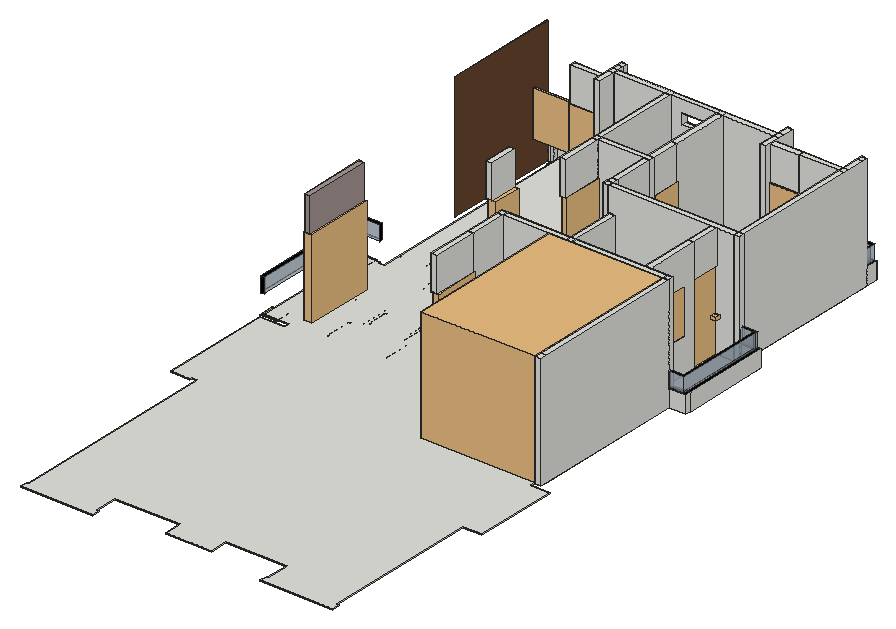
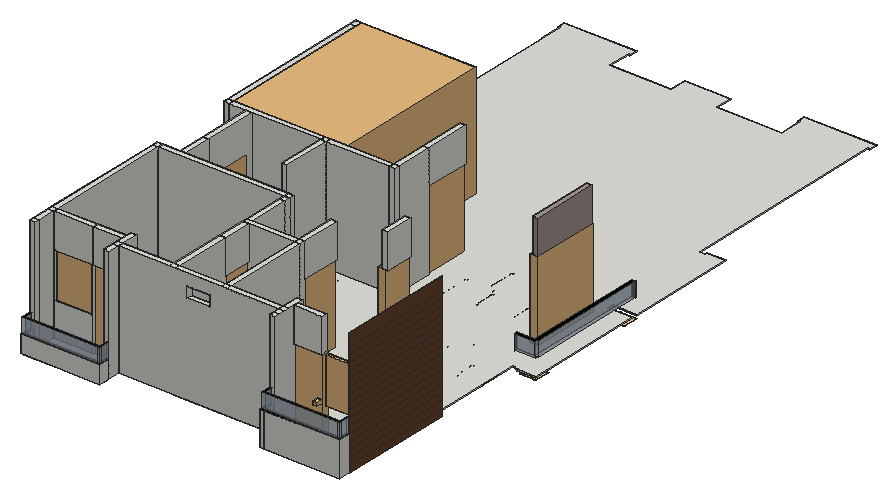
# SketchUp Ruby script. Lengths in inches.
U = 1.inch
M = Sketchup.active_model
def pt(a) = Geom::Point3d.new(a.map { |v| v * U })
def face(e, loops, mat)
  f = e.add_face(loops[0].map { |a| pt(a) })
  loops[1..].each { |l| e.add_face(l.map { |a| pt(a) }).erase! }
  f.material = f.back_material = mat if mat
  f
end
# faces: each face lists its corners as indices into pts; further lists are holes
def faces(e, pts, list, mat = nil) = list.each { |f| face(e, (f[0].is_a?(Array) ? f : [f]).map { |l| l.map { |i| pts[i] } }, mat) }
# xy, xz, yz: faces in a plane at the given z, y or x. An outline is a flat list of corners, or four numbers for a rectangle; further outlines are holes
def ring(l) = l.size == 4 ? [[l[0], l[1]], [l[2], l[1]], [l[2], l[3]], [l[0], l[3]]] : l.each_slice(2).to_a
def flat(e, list, mat, &to3) = list.each { |f| face(e, (f[0].is_a?(Array) ? f : [f]).map { |l| ring(l).map { |u, v| to3.(u, v) } }, mat) }
def xy(e, z, list, mat = nil) = flat(e, list, mat) { |x, y| [x, y, z] }
def xz(e, y, list, mat = nil) = flat(e, list, mat) { |x, z| [x, y, z] }
def yz(e, x, list, mat = nil) = flat(e, list, mat) { |y, z| [x, y, z] }
def lines(e, pts, list) = list.each { |a, b| e.add_line(pt(pts[a]), pt(pts[b])) }
# prism: a flat outline (further loops are holes) pulled along v
def prism(e, loops, v, mat = nil)
  f = face(e, loops, mat); d = Geom::Vector3d.new(v.map { |x| x * U })
  f.pushpull(f.normal.samedirection?(d) ? d.length : -d.length)
end
def box(e, o, s, mat = nil) = prism(e, [[o, [o[0] + s[0], o[1], o[2]], [o[0] + s[0], o[1] + s[1], o[2]], [o[0], o[1] + s[1], o[2]]]], [0, 0, s[2]], mat)
def at(x, y, z, deg = 0) = Geom::Transformation.translation(pt([x, y, z])) * Geom::Transformation.rotation(ORIGIN, Z_AXIS, deg.degrees)
def axes(o, x, y, z) = Geom::Transformation.new([*x, 0, *y, 0, *z, 0, *pt(o).to_a, 1])
def part(name) = M.definitions.add(name)
# library, detail: a bought-in or finely detailed component or shape, given as its bounding box
def library(name, o, s) = part(name).tap { |d| box(d.entities, o, s) }
def detail(e, o, s) = box(e.add_group.entities, o, s)
def put(e, d, t, mat = nil) = e.add_instance(d, t).tap { |i| i.material = mat if mat }
def group(e, t, mat = nil) = e.add_group.tap { |g| g.transformation = t; g.material = mat if mat }.entities
root = M.entities
M.materials.add("0-off white").color = [255, 255, 255]
M.materials.add("Glass_Basic_01").color = [161, 173, 186]
M.materials["Glass_Basic_01"].alpha = 0.59
M.materials.add("M09_Shadow_Night").color = [0, 0, 0]
M.materials.add("Marble_06_1K").color = [165, 150, 147]
M.materials.add("Wood_Veneer_15_1K").color = [103, 69, 45]
c1 = library("Return staircase",[0,-11.89,0],[120,168,120])
c2 = part("Group\#84")
xy(c2.entities,0,[[[-2,-32,-2,-24,0.04,-24,0.04,0,0,0,0,198,-6,198,-6,196,-25.9,196,-25.9,312.57,0,312.57,0,318.21,-25.9,318.21,-25.9,446,-6,446,-6,444,0,444,0,675.78,72,673.93,76,673.93,76,665.93,74,665.93,74,636,252.4,636,252.4,673.93,328.4,673.93,328.4,636,324.4,636,324.4,498.14,330.4,498.14,330.4,499.84,344.35,499.84,344.35,411,324.4,411,324.4,231,344.35,231,344.35,142,324.4,142,324.4,0,324.58,0,324.58,-24,326.4,-24,326.4,-32,250.4,-32,250.4,-24,252.4,-24,252.4,0,188.4,0,188.4,-18,140,-18,140,0,72,0,72,-24,74,-24,74,-32],[210.4,291,270.4,351]]])
xy(c2.entities,1,[[[-2,-32,74,-32,74,-24,72,-24,72,0,140,0,140,-18,188.4,-18,188.4,0,252.4,0,252.4,-24,250.4,-24,250.4,-32,326.4,-32,326.4,-24,324.58,-24,324.58,0,324.4,0,324.4,142,344.35,142,344.35,231,324.4,231,324.4,411,344.35,411,344.35,499.84,330.4,499.84,330.4,498.14,324.4,498.14,324.4,636,328.4,636,328.4,673.93,252.4,673.93,252.4,636,74,636,74,665.93,76,665.93,76,673.93,72,673.93,0,675.78,0,444,-6,444,-6,446,-25.9,446,-25.9,318.21,0,318.21,0,312.57,-25.9,312.57,-25.9,196,-6,196,-6,198,0,198,0,0,0.04,0,0.04,-24,-2,-24],[210.4,291,270.4,351]]])
xz(c2.entities,-32,[[-2,0,74,1],[250.4,0,326.4,1]])
xz(c2.entities,-24,[[-2,0,0.04,1],[72,0,74,1],[250.4,0,252.4,1],[324.58,0,326.4,1]])
xz(c2.entities,-18,[[140,0,188.4,1]])
xz(c2.entities,0,[[0,0,0.04,1],[72,0,140,1],[188.4,0,252.4,1],[324.4,0,324.58,1]])
xz(c2.entities,142,[[324.4,0,344.35,1]])
xz(c2.entities,196,[[-25.9,0,-6,1]])
xz(c2.entities,198,[[-6,0,0,1]])
xz(c2.entities,231,[[324.4,0,344.35,1]])
xz(c2.entities,291,[[210.4,0,270.4,1]])
xz(c2.entities,312.57,[[-25.9,0,0,1]])
xz(c2.entities,318.21,[[-25.9,0,0,1]])
xz(c2.entities,351,[[210.4,0,270.4,1]])
xz(c2.entities,411,[[324.4,0,344.35,1]])
xz(c2.entities,444,[[-6,0,0,1]])
xz(c2.entities,446,[[-25.9,0,-6,1]])
xz(c2.entities,498.14,[[324.4,0,330.4,1]])
xz(c2.entities,499.84,[[330.4,0,344.35,1]])
xz(c2.entities,636,[[74,0,252.4,1],[324.4,0,328.4,1]])
xz(c2.entities,665.93,[[74,0,76,1]])
xz(c2.entities,673.93,[[72,0,76,1],[252.4,0,328.4,1]])
yz(c2.entities,-25.9,[[196,0,312.57,1],[318.21,0,446,1]])
yz(c2.entities,-6,[[196,0,198,1],[444,0,446,1]])
yz(c2.entities,-2,[[-32,0,-24,1]])
yz(c2.entities,0,[[0,0,198,1],[312.57,0,318.21,1],[444,0,636,1],[636,0,637.85,1],[637.85,0,675.78,1]])
yz(c2.entities,0.04,[[-24,0,0,1]])
yz(c2.entities,72,[[-24,0,0,1]])
yz(c2.entities,74,[[-32,0,-24,1],[636,0,665.93,1]])
yz(c2.entities,76,[[665.93,0,673.93,1]])
yz(c2.entities,140,[[-18,0,0,1]])
yz(c2.entities,188.4,[[-18,0,0,1]])
yz(c2.entities,210.4,[[291,0,351,1]])
yz(c2.entities,250.4,[[-32,0,-24,1]])
yz(c2.entities,252.4,[[-24,0,0,1],[636,0,673.93,1]])
yz(c2.entities,270.4,[[291,0,351,1]])
yz(c2.entities,324.4,[[0,0,142,1],[231,0,411,1],[498.14,0,636,1]])
yz(c2.entities,324.58,[[-24,0,0,1]])
yz(c2.entities,326.4,[[-32,0,-24,1]])
yz(c2.entities,328.4,[[636,0,673.93,1]])
yz(c2.entities,330.4,[[498.14,0,499.84,1]])
yz(c2.entities,344.35,[[142,0,231,1],[411,0,499.84,1]])
# 3 loose lines left out
p = [[77.67,648,0],[77.67,636,1],[246.4,636,1],[246.4,648,0],[72,673.93,0],[0,675.78,0],
  [0,675.78,1],[72,673.93,1]]
faces(c2.entities,p,[[0,1,2,3],[4,5,6,7]])
c3 = library("TREE-26",[-60.96,-72.91,0],[121.92,134.74,0.01])
c4 = library("HYHHYHYHYHYHY",[-2.09,-4.54,0],[4.18,9.08,0.01])
c5 = library("Group\#51",[0,0,0],[6.9375,42,86.5])
c6 = part("feeeeeeeeee")
p = [[-2.68,3.51,0],[-2.68,3.16,0],[-2.92,3.16,0],[-2.92,3.07,0],[-3.56,3.07,0],[-3.56,3.51,0],
  [-2.68,-3.51,0],[-2.68,-3.16,0],[-2.92,-3.16,0],[-2.92,-3.07,0],[-3.56,-3.07,0],[-3.56,-3.51,0],
  [3.56,3.16,0],[-2.68,2.93,0],[3.56,2.93,0],[-2.48,-3.13,0],[-2.04,-3.07,0],[-1.61,-2.98,0],
  [-1.1875,-2.86,0],[-0.77,-2.72,0],[-0.36,-2.55,0],[0.03,-2.35,0],[0.41,-2.13,0],[0.78,-1.88,0],
  [1.125,-1.62,0],[1.46,-1.32,0],[1.77,-1.01,0],[2.06,-0.68,0],[2.33,-0.33,0],[2.57,0.03,0],
  [2.79,0.42,0],[2.99,0.81,0],[3.16,1.22,0],[3.3,1.63,0],[3.41,2.06,0],[3.5,2.49,0]]
lines(c6.entities,p,[[0,1],[1,2],[2,3],[3,4],[4,5],[5,0],[6,7],[7,8],[8,9],[9,10],[10,11],[11,6],
  [1,12],[13,14],[1,13],[12,14],[8,15],[15,16],[16,17],[17,18],[18,19],[19,20],[20,21],[21,22],
  [22,23],[23,24],[24,25],[25,26],[26,27],[27,28],[28,29],[29,30],[30,31],[31,32],[32,33],[33,34],
  [34,35],[35,14]])
c7 = part("Group\#305")
xy(c7.entities,0.81,[[0.28,-0.04,1.69,0]],"0-off white")
xz(c7.entities,-0.04,[[0.28,0.81,1.69,0.81,0.98,1.5]],"0-off white")
xz(c7.entities,0,[[[0.98,0,1.24,0.03,1.48,0.13,1.68,0.29,1.84,0.49,1.93,0.73,1.97,0.98,1.93,1.24,1.84,1.48,1.68,1.68,1.48,1.84,1.24,1.93,0.98,1.97,0.73,1.93,0.49,1.84,0.29,1.68,0.13,1.48,0.03,1.24,0,0.98,0.03,0.73,0.13,0.49,0.29,0.29,0.49,0.13,0.73,0.03],[0.28,0.81,0.98,1.5,1.69,0.81]]],"0-off white")
xz(c7.entities,0.63,[[0.98,0,0.73,0.03,0.49,0.13,0.29,0.29,0.13,0.49,0.03,0.73,0,0.98,0.03,1.24,0.13,1.48,0.29,1.68,0.49,1.84,0.73,1.93,0.98,1.97,1.24,1.93,1.48,1.84,1.68,1.68,1.84,1.48,1.93,1.24,1.97,0.98,1.93,0.73,1.84,0.49,1.68,0.29,1.48,0.13,1.24,0.03]],"0-off white")
p = [[0.49,0.63,0.13],[0.73,0.63,0.03],[0.73,0,0.03],[0.49,0,0.13],[0.98,0.63,0],[0.98,0,0],
  [1.24,0.63,0.03],[1.24,0,0.03],[1.48,0.63,0.13],[1.48,0,0.13],[0.29,0.63,0.29],[0.29,0,0.29],
  [1.68,0.63,0.29],[1.68,0,0.29],[0.13,0.63,0.49],[0.13,0,0.49],[1.84,0.63,0.49],[1.84,0,0.49],
  [0.03,0.63,0.73],[0.03,0,0.73],[1.93,0.63,0.73],[1.93,0,0.73],[0,0.63,0.98],[0,0,0.98],
  [1.97,0.63,0.98],[1.97,0,0.98],[0.98,0,1.5],[0.28,0,0.81],[0.28,-0.04,0.81],[0.98,-0.04,1.5],
  [1.69,0,0.81],[1.69,-0.04,0.81],[0.03,0.63,1.24],[0.03,0,1.24],[1.93,0.63,1.24],[1.93,0,1.24],
  [0.13,0.63,1.48],[0.13,0,1.48],[1.84,0.63,1.48],[1.84,0,1.48],[0.29,0.63,1.68],[0.29,0,1.68],
  [1.68,0.63,1.68],[1.68,0,1.68],[0.49,0.63,1.84],[0.49,0,1.84],[1.48,0.63,1.84],[1.48,0,1.84],
  [0.73,0.63,1.93],[0.73,0,1.93],[1.24,0.63,1.93],[1.24,0,1.93],[0.98,0.63,1.97],[0.98,0,1.97]]
faces(c7.entities,p,[[0,1,2,3],[1,4,5,2],[4,6,7,5],[6,8,9,7],[10,0,3,11],[8,12,13,9],[14,10,11,15],[12,16,17,13],
  [18,14,15,19],[16,20,21,17],[22,18,19,23],[20,24,25,21],[26,27,28,29],[30,26,29,31],[32,22,23,33],[24,34,35,25],
  [36,32,33,37],[34,38,39,35],[40,36,37,41],[38,42,43,39],[44,40,41,45],[42,46,47,43],[48,44,45,49],[46,50,51,47],
  [52,48,49,53],[50,52,53,51]],"0-off white")
c8 = part("Group\#370")
box(c8.entities,[0,0,-0.39],[5.12,10.31,0.39])
g1 = group(c8.entities,at(1.59,1.64,0.22))
put(g1,c7,axes([0,4.49,0],[1,0,0],[0,0,-0.35294],[0,1,0]))
put(g1,c7,axes([0,2,0],[1,0,0],[0,0,-0.35294],[0,-1,0]))
c9 = part("Group\#12")
xy(c9.entities,0,[[0,0,6,7.18],[0,7.18,6,168],[-174.4,129.21,-168.4,168],[-174.4,168,-168.4,174],[-168.4,168,-102,174],
  [-102,168,-96,174],[-96,168,0,174],[0,168,6,174],[6,168,24,174],[-102,174,-96,225]])
xy(c9.entities,18,[[6,168,24,174]],"M09_Shadow_Night")
xy(c9.entities,120,[[0,0,6,7.18],[0,7.18,6,168],[-174.4,129.21,-168.4,168],[-174.4,168,-168.4,174],[-168.4,168,-102,174],
  [-102,168,-96,174],[-96,168,0,174],[0,168,6,174],[-102,174,-96,225]])
xz(c9.entities,0,[[0,0,6,120]])
xz(c9.entities,129.21,[[-174.4,0,-168.4,120]])
xz(c9.entities,168,[[-174.4,0,-168.4,120],[-168.4,0,-102,120],[-102,0,-96,120],[-96,0,0,120],[0,0,6,120],
  [6,0,24,18]])
xz(c9.entities,174,[[-174.4,0,-168.4,120],[-168.4,0,-102,120],[-102,0,-96,120],[-96,0,0,120],[0,0,6,120],
  [6,0,24,18]])
xz(c9.entities,225,[[-102,0,-96,120]])
yz(c9.entities,-174.4,[[129.21,0,168,120],[168,0,174,120]])
yz(c9.entities,-168.4,[[129.21,0,168,120],[168,0,174,120]])
yz(c9.entities,-102,[[168,0,174,120],[174,0,225,120]])
yz(c9.entities,-96,[[168,0,174,120],[174,0,225,120]])
yz(c9.entities,0,[[0,0,7.18,120],[7.18,0,168,120],[168,0,174,120]])
yz(c9.entities,6,[[0,0,168,120],[168,0,174,18],[168,18,174,120]])
yz(c9.entities,24,[[168,0,174,18]])
c10 = library("porta correr aluminio",[0,0,0],[4.49,110.28,83.35])
c11 = library("VVVV",[-3.39,-3.68,0],[6.78,7.36,0.01])
c12 = library("BFGFV",[-4.32,-2.51,0],[8.64,5.02,0.01])
c13 = part("Group\#86")
xy(c13.entities,0,[[80,-8.86,82,2],[2,0,80,2]])
xy(c13.entities,16,[[80,-8.86,82,2],[2,0,80,2]],"M09_Shadow_Night")
xz(c13.entities,-8.86,[[80,0,82,16]],"M09_Shadow_Night")
xz(c13.entities,0,[[2,0,80,16]],"Glass_Basic_01")
xz(c13.entities,2,[[2,0,80,16]])
yz(c13.entities,2,[[0,0,2,16]],"M09_Shadow_Night")
yz(c13.entities,80,[[-8.86,0,0,16],[0,0,2,16]])
yz(c13.entities,82,[[-8.86,0,2,16]])
c14 = library("burner",[-300,-225,0],[600,450,0.01])
c15 = library("Slide Window 5'",[0,-2.02,0],[60,2.02,54])
c16 = library("lcd-01",[-577.99,-134.75,0],[1155.98,269.5,0.01])
c17 = part("Component\#5")
p = [[1166.02,522.1,0],[1167.27,522.1,0],[1183.11,522.1,0],[1183.72,522.1,0],[1165.72,517.1,0],[1167.27,517.1,0],
  [1183.11,517.1,0],[1183.72,517.1,0],[1165.72,512.1,0],[1167.27,512.1,0],[1183.11,512.1,0],[1183.72,512.1,0],
  [1165.72,507.1,0],[1167.27,507.1,0],[1183.11,507.1,0],[1183.72,507.1,0],[1165.72,502.1,0],[1167.27,502.1,0],
  [1183.11,502.1,0],[1183.72,502.1,0],[1165.72,497.1,0],[1167.27,497.1,0],[1183.11,497.1,0],[1183.72,497.1,0],
  [1165.72,492.1,0],[1183.72,492.1,0],[1165.72,487.1,0],[1183.72,487.1,0],[1111.72,482.1,0],[1128.65,482.1,0],
  [1150.05,482.1,0],[1183.72,482.1,0],[1111.72,477.1,0],[1128.65,477.1,0],[1150.05,477.1,0],[1183.72,477.1,0],
  [1111.72,472.1,0],[1128.65,472.1,0],[1150.05,472.1,0],[1173.72,472.1,0],[1117.28,469.6,0],[1112.28,474.6,0],
  [1127.28,479.6,0],[1122.28,484.6,0],[1157.28,469.6,0],[1152.28,474.6,0],[1173.72,473.16,0],[1172.28,474.6,0],
  [1167.28,479.6,0],[1162.28,484.6,0],[1183.72,483.16,0],[1182.28,484.6,0],[1177.28,489.6,0],[1172.48,494.4,0],
  [1167.27,499.61,0],[1165.72,501.16,0],[1183.72,503.16,0],[1183.11,503.77,0],[1167.27,519.61,0],[1165.77,521.11,0],
  [1183.72,523.16,0],[1182.3,524.58,0],[1118.53,469.6,0],[1113.53,474.6,0],[1128.53,479.6,0],[1123.53,484.6,0],
  [1158.53,469.6,0],[1153.53,474.6,0],[1173.72,474.41,0],[1173.53,474.6,0],[1168.53,479.6,0],[1163.53,484.6,0],
  [1183.72,484.41,0],[1183.53,484.6,0],[1178.53,489.6,0],[1173.73,494.4,0],[1167.27,500.86,0],[1165.72,502.41,0],
  [1183.72,504.41,0],[1183.53,504.6,0],[1167.27,520.86,0],[1166.02,522.11,0],[1183.72,524.41,0],[1183.55,524.58,0],
  [1119.78,469.6,0],[1114.78,474.6,0],[1128.65,480.73,0],[1124.78,484.6,0],[1159.78,469.6,0],[1154.78,474.6,0],
  [1169.78,479.6,0],[1164.78,484.6,0],[1179.78,489.6,0],[1174.98,494.4,0],[1167.27,502.11,0],[1165.72,503.66,0],
  [1167.27,522.11,0],[1166.48,522.9,0]]
lines(c17.entities,p,[[0,1],[2,3],[4,5],[6,7],[8,9],[10,11],[12,13],[14,15],[16,17],[18,19],[20,21],[22,23],
  [24,25],[26,27],[28,29],[30,31],[32,33],[34,35],[36,37],[38,39],[40,41],[42,43],[44,45],[46,47],
  [48,49],[50,51],[52,53],[54,55],[56,57],[58,59],[60,61],[62,63],[64,65],[66,67],[68,69],[70,71],
  [72,73],[74,75],[76,77],[78,79],[80,81],[82,83],[84,85],[86,87],[88,89],[90,91],[92,93],[94,95],
  [96,97]])
c18 = library("sink",[-449.92,-250,0],[899.84,500,0.01])
c19 = library("A$C72E23588",[-1177.7,-903.95,0],[2355.4,1807.9,0.01])
c20 = part("Group\#85")
xy(c20.entities,0,[[0,0,0,11.0625,2,11.0625,2,2,80,2,80,0],[80,0,82,2],[80,2,82,11.0625]])
xy(c20.entities,16,[[0,0,80,0,80,2,2,2,2,11.0625,0,11.0625],[80,0,82,2],[80,2,82,11.0625]],"M09_Shadow_Night")
xz(c20.entities,0,[[80,0,82,16]])
xz(c20.entities,0,[[0,0,80,16]],"Glass_Basic_01")
xz(c20.entities,2,[[2,0,80,16],[80,0,82,16]])
xz(c20.entities,11.0625,[[0,0,2,16],[80,0,82,16]])
yz(c20.entities,0,[[0,0,11.0625,16]])
yz(c20.entities,2,[[2,0,11.0625,16]])
yz(c20.entities,80,[[0,0,2,16],[2,0,11.0625,16]])
yz(c20.entities,82,[[0,0,2,16],[2,0,11.0625,16]])
c21 = part("Group\#14")
xy(c21.entities,0,[[0,0,4.05,3.45],[0,3.45,4.05,88.84],[-13.95,88.84,0,93],[0,88.84,4.05,93]])
xy(c21.entities,18,[[0,0,4.05,88.84],[-13.95,88.84,0,93],[0,88.84,4.05,93]],"M09_Shadow_Night")
xz(c21.entities,0,[[0,0,4.05,18]])
xz(c21.entities,88.84,[[-13.95,0,0,18]])
xz(c21.entities,93,[[-13.95,0,4.05,18]])
yz(c21.entities,-13.95,[[88.84,0,93,18]])
yz(c21.entities,0,[[0,0,3.45,18],[3.45,0,88.84,18]])
yz(c21.entities,4.05,[[0,0,93,18]])
c22 = library("JEEW",[-211.14,-299.86,0],[422.28,599.72,0.01])
c23 = library("ghgjg",[-265.23,-341.01,0],[530.46,682.02,0.01])
c24 = part("tgr")
p = [[-2.37,-3.35,0],[-2.37,-2.82,0],[-2.73,-2.82,0],[-2.73,-2.68,0],[-3.71,-2.68,0],[-3.71,-3.35,0],
  [-2.37,3.35,0],[-2.37,2.82,0],[-2.73,2.82,0],[-2.73,2.68,0],[-3.71,2.68,0],[-3.71,3.35,0],
  [3.71,-2.82,0],[-2.37,-2.46,0],[3.71,-2.46,0],[3.7,-2.46,0],[3.63,-2.07,0],[3.53,-1.68,0],
  [3.41,-1.3,0],[3.27,-0.93,0],[3.1,-0.57,0],[2.91,-0.22,0],[2.7,0.12,0],[2.46,0.4375,0],
  [2.21,0.74,0],[1.93,1.03,0],[1.64,1.3,0],[1.33,1.55,0],[1.01,1.79,0],[0.67,1.99,0],
  [0.32,2.18,0],[-0.04,2.35,0],[-0.41,2.49,0],[-0.8,2.6,0],[-1.18,2.69,0],[-1.58,2.76,0],
  [-1.97,2.8,0]]
lines(c24.entities,p,[[0,1],[1,2],[2,3],[3,4],[4,5],[5,0],[6,7],[7,8],[8,9],[9,10],[10,11],[11,6],
  [1,12],[13,14],[1,13],[12,14],[15,16],[16,17],[17,18],[18,19],[19,20],[20,21],[21,22],[22,23],
  [23,24],[24,25],[25,26],[26,27],[27,28],[28,29],[29,30],[30,31],[31,32],[32,33],[33,34],[34,35],
  [35,36],[36,7]])
c25 = library("Group\#49",[0,0,0],[8.31,30,84])
c26 = library("Group\#52",[0,0,0],[4.66,6.14,3.22])
c27 = part("EGWF")
p = [[2.59,-3.49,0],[2.59,-3.09,0],[2.85,-3.09,0],[2.85,-2.99,0],[3.58,-2.99,0],[3.58,-3.49,0],
  [2.59,3.49,0],[2.59,3.09,0],[2.85,3.09,0],[2.85,2.99,0],[3.58,2.99,0],[3.58,3.49,0],
  [-3.58,-3.09,0],[2.59,-2.82,0],[-3.58,-2.82,0],[2.2,3.07,0],[1.81,3.04,0],[1.42,2.97,0],
  [1.03,2.89,0],[0.66,2.78,0],[0.29,2.64,0],[-0.07,2.48,0],[-0.42,2.3,0],[-0.76,2.1,0],
  [-1.08,1.875,0],[-1.39,1.63,0],[-1.68,1.37,0],[-1.96,1.09,0],[-2.21,0.79,0],[-2.45,0.48,0],
  [-2.67,0.15,0],[-2.86,-0.1875,0],[-3.04,-0.54,0],[-3.1875,-0.9,0],[-3.32,-1.28,0],[-3.42,-1.66,0],
  [-3.5,-2.04,0],[-3.55,-2.43,0]]
lines(c27.entities,p,[[0,1],[1,2],[2,3],[3,4],[4,5],[5,0],[6,7],[7,8],[8,9],[9,10],[10,11],[11,6],
  [1,12],[13,14],[1,13],[12,14],[7,15],[15,16],[16,17],[17,18],[18,19],[19,20],[20,21],[21,22],
  [22,23],[23,24],[24,25],[25,26],[26,27],[27,28],[28,29],[29,30],[30,31],[31,32],[32,33],[33,34],
  [34,35],[35,36],[36,37],[37,14]])
c28 = library("double bed",[-999.9375,-1062.5,0],[1999.875,2125,0.01])
c29 = part("Group\#126")
xy(c29.entities,0,[[-138,-162.42,-132,-156.42],[-132,-162.42,0,-156.42],[0,-162.42,6,-156.42],[-138,-156.42,-132,-150.42],[0,-156.42,6,-24.42],
  [-42,-24.42,0,-18.42],[0,-24.42,6,-18.42],[0,-18.42,6,0],[0,0,6,5.51]])
xy(c29.entities,36,[[-40,-24.42,-2,-18.42]])
xy(c29.entities,84,[[-40,-24.42,-2,-18.42]])
xy(c29.entities,120,[[-138,-162.42,-132,-156.42],[-132,-162.42,0,-156.42],[0,-162.42,6,-156.42],[-138,-156.42,-132,-150.42],[0,-156.42,6,-24.42],
  [-42,-24.42,0,-18.42],[0,-24.42,6,-18.42],[0,-18.42,6,0],[0,0,6,5.51]])
xz(c29.entities,-162.42,[[-138,0,-132,120],[-132,0,0,120],[0,0,6,120]])
xz(c29.entities,-156.42,[[-138,0,-132,120],[-132,0,0,120],[0,0,6,120]])
xz(c29.entities,-150.42,[[-138,0,-132,120]])
xz(c29.entities,-24.42,[[[-42,0,0,120],[-40,36,-2,84]]])
xz(c29.entities,-18.42,[[[-42,0,0,120],[-40,36,-2,84]]])
xz(c29.entities,5.51,[[0,0,6,120]])
yz(c29.entities,-138,[[-162.42,0,-156.42,120],[-156.42,0,-150.42,120]])
yz(c29.entities,-132,[[-162.42,0,-156.42,120],[-156.42,0,-150.42,120]])
yz(c29.entities,-42,[[-24.42,0,-18.42,120]])
yz(c29.entities,-40,[[-24.42,36,-18.42,84]])
yz(c29.entities,-2,[[-24.42,36,-18.42,84]])
yz(c29.entities,0,[[-162.42,0,-156.42,120],[-156.42,0,-24.42,120],[-24.42,0,-18.42,120],[-18.42,0,0,120],[0,0,5.51,120]])
yz(c29.entities,6,[[-162.42,0,-156.42,120],[-156.42,0,5.51,120]])
c30 = part("Group\#116")
xy(c30.entities,0,[[24,0,24.75,24.75]])
xy(c30.entities,107,[[24,0,24.75,24.75]])
xz(c30.entities,0,[[24,0,24.75,107]])
xz(c30.entities,24.75,[[24,0,24.75,107]])
yz(c30.entities,24,[[0,0,24.75,6],[0,6,24.75,12],[0,12,24.75,18],[0,18,24.75,24],[0,24,24.75,30],
  [0,30,24.75,36],[0,36,24.75,42],[0,42,24.75,48],[0,48,24.75,54],[0,54,24.75,60],
  [0,60,24.75,66],[0,66,24.75,72],[0,72,24.75,78],[0,78,24.75,84],[0,84,24.75,90],
  [0,90,24.75,96],[0,96,24.75,107]],"Wood_Veneer_15_1K")
yz(c30.entities,24.75,[[0,0,24.75,107]])
c31 = part("G5GTGTGT")
p = [[0.52,4.97,0],[0.52,-4.97,0],[0.36,-4.97,0],[0.36,4.97,0],[-0.08,-4.53,0],[-0.08,4.53,0],
  [0.33,4.97,0],[0.3,4.97,0],[0.28,4.96,0],[0.25,4.96,0],[0.22,4.95,0],[0.2,4.94,0],
  [0.17,4.93,0],[0.15,4.92,0],[0.12,4.9,0],[0.1,4.89,0],[0.08,4.87,0],[0.06,4.85,0],
  [0.04,4.83,0],[0.02,4.8125,0],[0,4.79,0],[-0.01,4.77,0],[-0.03,4.74,0],[-0.04,4.72,0],
  [-0.05,4.69,0],[-0.0625,4.67,0],[-0.07,4.64,0],[-0.08,4.61,0],[-0.08,4.59,0],[-0.08,4.56,0],
  [-0.08,-4.56,0],[-0.08,-4.59,0],[-0.08,-4.61,0],[-0.07,-4.64,0],[-0.0625,-4.67,0],[-0.05,-4.69,0],
  [-0.04,-4.72,0],[-0.03,-4.74,0],[-0.01,-4.77,0],[0,-4.79,0],[0.02,-4.8125,0],[0.04,-4.83,0],
  [0.06,-4.85,0],[0.08,-4.87,0],[0.1,-4.89,0],[0.12,-4.9,0],[0.15,-4.92,0],[0.17,-4.93,0],
  [0.2,-4.94,0],[0.22,-4.95,0],[0.25,-4.96,0],[0.28,-4.96,0],[0.3,-4.97,0],[0.33,-4.97,0],
  [-0.08,-1.38,0],[-0.52,-1.38,0],[-0.08,1.38,0],[-0.52,1.38,0]]
lines(c31.entities,p,[[0,1],[1,2],[2,3],[3,0],[4,5],[3,6],[6,7],[7,8],[8,9],[9,10],[10,11],[11,12],
  [12,13],[13,14],[14,15],[15,16],[16,17],[17,18],[18,19],[19,20],[20,21],[21,22],[22,23],[23,24],
  [24,25],[25,26],[26,27],[27,28],[28,29],[29,5],[4,30],[30,31],[31,32],[32,33],[33,34],[34,35],
  [35,36],[36,37],[37,38],[38,39],[39,40],[40,41],[41,42],[42,43],[43,44],[44,45],[45,46],[46,47],
  [47,48],[48,49],[49,50],[50,51],[51,52],[52,53],[53,2],[54,55],[56,57],[55,57]])
c32 = part("Group\#15")
xy(c32.entities,0,[[60,-108.67,66,-102.67],[66,-108.67,120.4,-102.67],[60,-102.67,66,-12.67],[114.4,-72.67,120.4,-12.67],[0,-30.67,6,-12.67],
  [174.4,-30.67,180.4,-12.67],[0,-12.67,6,-6.67],[6,-12.67,60,-6.67],[60,-12.67,66,-6.67],[66,-12.67,114.4,-6.67],
  [114.4,-12.67,120.4,-6.67],[120.4,-12.67,174.4,-6.67],[174.4,-12.67,180.4,-6.67],[0,-6.67,6,0],[174.4,-6.67,180.4,5.26],
  [0,0,6,5.26]])
xy(c32.entities,96,[[78,-12.67,102.4,-6.67]])
xy(c32.entities,108,[[78,-12.67,102.4,-6.67]])
xy(c32.entities,120,[[60,-108.67,66,-102.67],[66,-108.67,120.4,-102.67],[60,-102.67,66,-12.67],[114.4,-72.67,120.4,-12.67],[0,-30.67,6,-12.67],
  [174.4,-30.67,180.4,-12.67],[0,-12.67,6,-6.67],[6,-12.67,60,-6.67],[60,-12.67,66,-6.67],[66,-12.67,114.4,-6.67],
  [114.4,-12.67,120.4,-6.67],[120.4,-12.67,174.4,-6.67],[174.4,-12.67,180.4,-6.67],[0,-6.67,6,0],[174.4,-6.67,180.4,5.26],
  [0,0,6,5.26]])
xz(c32.entities,-108.67,[[60,0,66,120],[66,0,120.4,120]])
xz(c32.entities,-102.67,[[60,0,66,120],[66,0,120.4,120]])
xz(c32.entities,-72.67,[[114.4,0,120.4,120]])
xz(c32.entities,-30.67,[[0,0,6,120],[174.4,0,180.4,120]])
xz(c32.entities,-12.67,[[6,0,60,120],[60,0,66,120],[[66,0,114.4,120],[78,96,102.4,108]],[114.4,0,120.4,120],[120.4,0,174.4,120]])
xz(c32.entities,-6.67,[[[6,0,174.4,120],[78,96,102.4,108]]])
xz(c32.entities,5.26,[[0,0,6,120],[174.4,0,180.4,120]])
yz(c32.entities,0,[[-30.67,0,5.26,120]])
yz(c32.entities,6,[[-30.67,0,-12.67,120],[-12.67,0,-6.67,120],[-6.67,0,0,120],[0,0,5.26,120]])
yz(c32.entities,60,[[-108.67,0,-102.67,120],[-102.67,0,-12.67,120]])
yz(c32.entities,66,[[-108.67,0,-102.67,120],[-102.67,0,-12.67,120]])
yz(c32.entities,78,[[-12.67,96,-6.67,108]])
yz(c32.entities,102.4,[[-12.67,96,-6.67,108]])
yz(c32.entities,114.4,[[-72.67,0,-12.67,120]])
yz(c32.entities,120.4,[[-108.67,0,-102.67,120],[-72.67,0,-12.67,120]])
yz(c32.entities,174.4,[[-30.67,0,-12.67,120],[-12.67,0,-6.67,120],[-6.67,0,5.26,120]])
yz(c32.entities,180.4,[[-30.67,0,5.26,120]])
c33 = library("Group\#48",[0,0,0],[6.9375,42,86.5])
c34 = library("Component\#3",[961.32,686.58,0],[54,18,0.01])
c35 = library("Component\#4",[1075.72,686.58,0],[54,18,0.01])
c36 = part("Group\#90")
xy(c36.entities,0,[[0,0,0,11.0625,2,11.0625,2,2,80,2,80,0],[80,0,82,2],[80,2,82,11.0625]])
xy(c36.entities,16,[[0,0,80,0,80,2,2,2,2,11.0625,0,11.0625],[80,0,82,2],[80,2,82,11.0625]],"M09_Shadow_Night")
xz(c36.entities,0,[[80,0,82,16]])
xz(c36.entities,0,[[0,0,80,16]],"Glass_Basic_01")
xz(c36.entities,2,[[2,0,80,16],[80,0,82,16]])
xz(c36.entities,11.0625,[[0,0,2,16],[80,0,82,16]])
yz(c36.entities,0,[[0,0,11.0625,16]])
yz(c36.entities,2,[[2,0,11.0625,16]])
yz(c36.entities,80,[[0,0,2,16],[2,0,11.0625,16]])
yz(c36.entities,82,[[0,0,2,16],[2,0,11.0625,16]])
c37 = part("Group\#16")
xy(c37.entities,0,[[0,0,4,3.74],[80,0,84,8],[0,3.74,4,8],[0,8,4,12],[4,8,80,12],
  [80,8,84,12]])
xy(c37.entities,18,[[0,0,4,12],[80,0,84,0,84,12,4,12,4,8,80,8]],"M09_Shadow_Night")
xz(c37.entities,0,[[0,0,4,18],[80,0,84,18]])
xz(c37.entities,8,[[4,0,80,18]])
xz(c37.entities,12,[[0,0,84,18]])
yz(c37.entities,0,[[0,0,12,18]])
yz(c37.entities,4,[[0,0,3.74,18],[3.74,0,8,18]])
yz(c37.entities,80,[[0,0,8,18]])
yz(c37.entities,84,[[0,0,12,18]])
c38 = part("Group\#13")
xy(c38.entities,0,[[0,0,4,3.01],[80,0,84,8],[0,3.01,4,8],[0,8,4,12],[4,8,80,12],
  [80,8,84,12]])
xy(c38.entities,36,[[0,0,4,12],[80,0,84,12],[4,8,80,12]],"M09_Shadow_Night")
xz(c38.entities,0,[[0,0,4,36],[80,0,84,36]])
xz(c38.entities,8,[[4,0,80,36]])
xz(c38.entities,12,[[0,0,80,36],[80,0,84,36]])
yz(c38.entities,0,[[0,0,12,36]])
yz(c38.entities,4,[[0,0,3.01,36],[3.01,0,8,36]])
yz(c38.entities,80,[[0,0,8,36],[8,0,12,36]])
yz(c38.entities,84,[[0,0,12,36]])
box(root,[181.8,391.55,204],[6,48,36])
box(root,[37.8,404.89,204],[6,71.14,36],"Marble_06_1K")
prism(root,[[[338.2,484.34,120],[338.2,541.34,120],[338.2,541.34,240],[338.2,484.34,240]],[[338.2,490.34,156],[338.2,490.34,204],[338.2,529.34,204],[338.2,529.34,156]]],[-6,0,0])
box(root,[332.19,541.34,204],[6.01,30,36])
box(root,[119.8,541.34,204],[6,30,36])
box(root,[218.2,583.34,204],[6,42,36])
box(root,[163.8,583.34,204],[6,42,36])
box(root,[218.2,631.34,204],[6,30,36])
box(root,[284.2,709.34,204],[30,6,36])
box(root,[73.8,709.34,204],[30,6,36])
box(root,[224.2,703.34,120],[54,18,1])
xy(root,120,[[218.2,571.34,362.2,571.34,362.2,739.27,356.2,739.27,356.2,715.34,314.2,715.34,314.2,709.34,356.2,709.34,356.2,577.34,224.2,577.34,224.2,583.34,218.2,583.34]])
put(root,c1,at(236.2,322.23,120))
put(root,c2,at(31.8,73.34,120))
put(root,c3,axes([12.58,398.13,120],[0,0.1317,0],[0.1317,0,0],[0,0,0.1317]))
put(root,c4,axes([99.08,410.24,120],[0,-6.75189,0],[6.75189,0,0],[0,0,6.75189]))
put(root,c5,axes([189.46,439.01,120],[-0.85622,0,0],[0,-1.13,0],[0,0,0.9711]))
put(root,c6,axes([163.46,415.55,120],[-6.83664,0,0],[0,-6.83664,0],[0,0,6.83664]))
put(root,c8,axes([236.2,421.93,170.05],[0,-0.53664,0],[0,0,1],[-1.59369,0,0]))
put(root,c9,at(356.2,310.34,120))
put(root,c10,axes([45.93,404.95,120.65],[-1.89519,0,0],[0,0.65291,0],[0,0,1]))
put(root,c11,axes([138,443.33,120],[-4.47564,0,0],[0,4.47564,0],[0,0,4.47564]))
put(root,c11,axes([64.42,443.33,120],[4.47564,0,0],[0,4.47564,0],[0,0,4.47564]))
put(root,c12,axes([101.4,444.26,120],[4.3395,0,0],[0,4.3395,0],[0,0,4.3395]))
put(root,c13,axes([6.91,388.28,140],[0,1.63485,0],[-2.08447,0,0],[0,0,1]),"Glass_Basic_01")
put(root,c3,axes([371.8,491.09,120],[0,0.1317,0],[0.1317,0,0],[0,0,0.1317]))
put(root,c14,axes([287.83,493.58,120],[-0.03566,0,0],[0,-0.03566,0],[0,0,0.03566]))
put(root,c15,axes([336.93,529.39,155.94],[0,-0.65094,0],[1.4091,0,0],[0,0,0.88889]))
put(root,c16,axes([102.68,511.95,120],[0.04,0,0],[0,0.04,0],[0,0,0.04]))
put(root,c17,at(-851.52,16.76,120))
put(root,c3,axes([12.58,513.99,120],[0,0.1317,0],[0.1317,0,0],[0,0,0.1317]))
put(root,c18,axes([323.67,525.41,120],[0,0.03168,0],[0.03168,0,0],[0,0,0.03168]))
put(root,c19,axes([191.83,525.47,120],[0.0356,0,0],[0,-0.0356,0],[0,0,0.0356]))
put(root,c20,axes([377.67,479.34,138],[0,1.18,0],[-1.39867,0,0],[0,0,1]),"Glass_Basic_01")
put(root,c21,at(376.15,484.34,120))
put(root,c22,axes([106.95,532.38,120],[0,-0.04284,0],[-0.04284,0,0],[0,0,0.04284]))
put(root,c23,axes([45.4375,547.34,120],[0,-0.04,0],[-0.04,0,0],[0,0,0.04]))
put(root,c24,axes([348.8,556.34,120],[4.47464,0,0],[0,-4.47464,0],[0,0,4.47464]))
put(root,c5,axes([330.54,541.34,120],[0.85622,0,0],[0,0.71429,0],[0,0,0.9711]))
put(root,c24,axes([109.2,556.34,120],[-4.47464,0,0],[0,-4.47464,0],[0,0,4.47464]))
put(root,c25,at(121.52,541.34,120))
put(root,c26,at(336.48,569.34,156.75,-90))
put(root,c3,axes([371.8,567.61,120],[0,0.1317,0],[0.1317,0,0],[0,0,0.1317]))
put(root,c27,axes([239.8,604.34,120],[-6.02515,0,0],[0,6.02515,0],[0,0,6.02515]))
put(root,c27,axes([148.2,604.34,120],[6.02515,0,0],[0,6.02515,0],[0,0,6.02515]))
put(root,c25,axes([222.48,625.34,120],[-1,0,0],[0,-1.4,0],[0,0,1]))
put(root,c5,axes([171.46,625.34,120],[-0.85622,0,0],[0,-1,0],[0,0,0.9711]))
put(root,c28,axes([71.06,633.07,120],[0,-0.03695,0],[-0.03695,0,0],[0,0,0.03695]))
put(root,c28,axes([316.9375,633.07,120],[0,-0.03695,0],[0.03695,0,0],[0,0,0.03695]))
put(root,c22,axes([178.84,644.18,120],[-0.04284,0,0],[0,0.04284,0],[0,0,0.04284]))
put(root,c24,axes([207.6,646.34,120],[-4.47464,0,0],[0,4.47464,0],[0,0,4.47464]))
put(root,c5,axes([225.86,661.34,120],[-0.85622,0,0],[0,-0.71429,0],[0,0,0.9711]))
put(root,c16,axes([158.41,652,120],[0,-0.04,0],[0.04,0,0],[0,0,0.04]))
put(root,c29,at(356.2,733.76,120))
put(root,c30,axes([1.05,618.07,120],[1,0,0],[0,4.89695,0],[0,0,1.23364]),"Wood_Veneer_15_1K")
put(root,c31,axes([226.1,681.76,120],[3.62,0,0],[0,3.62,0],[0,0,3.62]))
put(root,c32,at(103.8,734.01,120))
put(root,c23,axes([193.9,707.6,120],[-0.04,0,0],[0,0.04,0],[0,0,0.04]))
put(root,c5,axes([103.8,707.68,120],[0,0.85622,0],[-0.71429,0,0],[0,0,0.97071]))
put(root,c33,axes([314.2,707.68,120],[0,0.85622,0],[-0.71429,0,0],[0,0,0.97071]))
put(root,c15,axes([316.2,713.15,156],[0.63333,0,0],[0,1.4091,0],[0,0,0.88889]))
put(root,c15,axes([33.8,713.23,156],[0.63333,0,0],[0,1.4091,0],[0,0,0.88889]))
put(root,c34,at(-851.52,16.76,120))
put(root,c35,at(-851.52,16.76,120))
put(root,c26,at(287.63,713.62,156.75))
put(root,c26,at(75.08,713.8,156.89))
put(root,c24,axes([299.2,725.9375,120],[0,4.47464,0],[4.47464,0,0],[0,0,4.47464]))
put(root,c24,axes([88.8,725.9375,120],[0,4.47464,0],[-4.47464,0,0],[0,0,4.47464]))
put(root,c3,axes([38.7,741.86,120],[0,0.1317,0],[0.1317,0,0],[0,0,0.1317]))
put(root,c3,axes([349.66,741.86,120],[0,0.1317,0],[0.1317,0,0],[0,0,0.1317]))
put(root,c36,at(361.2,750.33,138,180),"Glass_Basic_01")
put(root,c36,at(108.8,750.33,156,180),"Glass_Basic_01")
put(root,c37,at(278.2,739.27,120))
put(root,c38,at(25.8,739.27,120))
